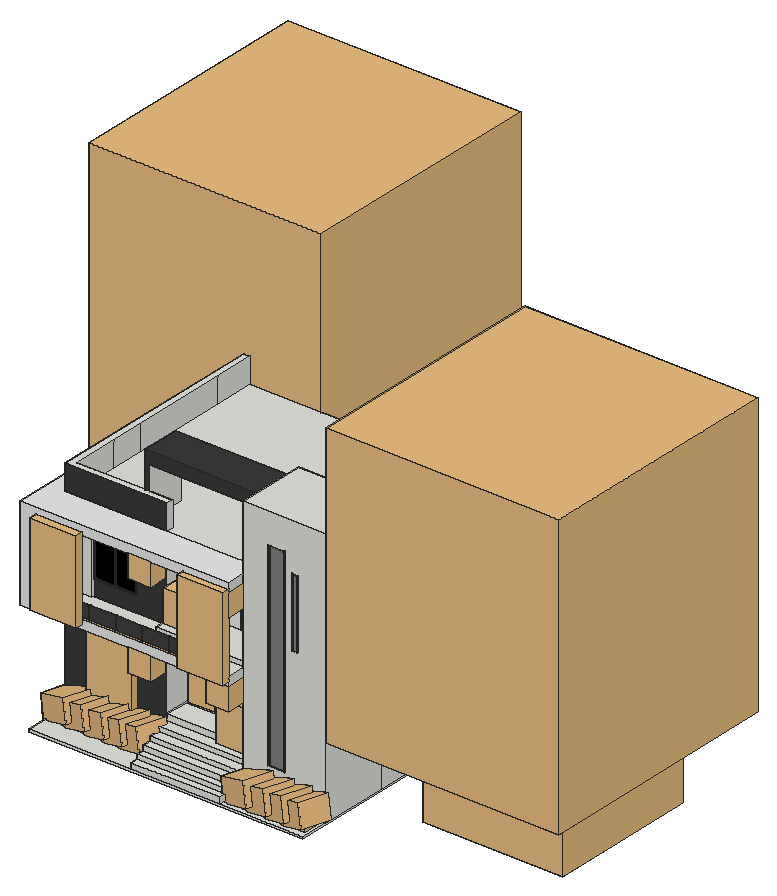
# SketchUp Ruby script. Lengths in inches.
U = 1.inch
M = Sketchup.active_model
def pt(a) = Geom::Point3d.new(a.map { |v| v * U })
def face(e, loops, mat)
  f = e.add_face(loops[0].map { |a| pt(a) })
  loops[1..].each { |l| e.add_face(l.map { |a| pt(a) }).erase! }
  f.material = f.back_material = mat if mat
  f
end
# faces: each face lists its corners as indices into pts; further lists are holes
def faces(e, pts, list, mat = nil) = list.each { |f| face(e, (f[0].is_a?(Array) ? f : [f]).map { |l| l.map { |i| pts[i] } }, mat) }
# xy, xz, yz: faces in a plane at the given z, y or x. An outline is a flat list of corners, or four numbers for a rectangle; further outlines are holes
def ring(l) = l.size == 4 ? [[l[0], l[1]], [l[2], l[1]], [l[2], l[3]], [l[0], l[3]]] : l.each_slice(2).to_a
def flat(e, list, mat, &to3) = list.each { |f| face(e, (f[0].is_a?(Array) ? f : [f]).map { |l| ring(l).map { |u, v| to3.(u, v) } }, mat) }
def xy(e, z, list, mat = nil) = flat(e, list, mat) { |x, y| [x, y, z] }
def xz(e, y, list, mat = nil) = flat(e, list, mat) { |x, z| [x, y, z] }
def yz(e, x, list, mat = nil) = flat(e, list, mat) { |y, z| [x, y, z] }
def lines(e, pts, list) = list.each { |a, b| e.add_line(pt(pts[a]), pt(pts[b])) }
# prism: a flat outline (further loops are holes) pulled along v
def prism(e, loops, v, mat = nil)
  f = face(e, loops, mat); d = Geom::Vector3d.new(v.map { |x| x * U })
  f.pushpull(f.normal.samedirection?(d) ? d.length : -d.length)
end
def box(e, o, s, mat = nil) = prism(e, [[o, [o[0] + s[0], o[1], o[2]], [o[0] + s[0], o[1] + s[1], o[2]], [o[0], o[1] + s[1], o[2]]]], [0, 0, s[2]], mat)
def at(x, y, z, deg = 0) = Geom::Transformation.translation(pt([x, y, z])) * Geom::Transformation.rotation(ORIGIN, Z_AXIS, deg.degrees)
def axes(o, x, y, z) = Geom::Transformation.new([*x, 0, *y, 0, *z, 0, *pt(o).to_a, 1])
def part(name) = M.definitions.add(name)
# library, detail: a bought-in or finely detailed component or shape, given as its bounding box
def library(name, o, s) = part(name).tap { |d| box(d.entities, o, s) }
def detail(e, o, s) = box(e.add_group.entities, o, s)
def put(e, d, t, mat = nil) = e.add_instance(d, t).tap { |i| i.material = mat if mat }
def group(e, t, mat = nil) = e.add_group.tap { |g| g.transformation = t; g.material = mat if mat }.entities
root = M.entities
M.materials.add("AM113_062_Tilia").color = [58, 81, 37]
M.materials.add("AM113_062_Tilia_Bark").color = [88, 85, 72]
M.materials.add("Glass_Tinted_Gray").color = [0, 0, 0]
M.materials.add("Material__1").color = [190, 136, 85]
M.materials.add("Material__2").color = [51, 42, 44]
M.materials.add("Material__3").color = [119, 136, 107]
M.materials.add("[0135_DarkGray]").color = [81, 81, 81]
M.materials.add("[Color M07]").color = [58, 58, 58]
M.materials.add("[Mirror 02]").color = [229, 229, 229]
M.materials.add("[Terrazzo Light Blue]").color = [196, 214, 227]
M.materials.add("[Translucent Glass Gray]1").color = [128, 128, 128]
M.materials.add("[Translucent_Glass_Blue]").color = [63, 63, 63]
M.materials.add("metal railing").color = [165, 165, 165]
M.materials.add("plastic2").color = [86, 86, 86]
M.materials.add("white_wall").color = [233, 233, 233]
c1 = library("PINTU+6+YA",[0,-0.6875,0],[35.83,8.07,80.71])
c2 = part("Window (2)")
xy(c2.entities,31.72,[[-0.78,88.6,2.72,128.1]])
xy(c2.entities,34.95,[[-0.78,91.53,0.84,106.59],[0.84,91.53,1.05,97.58],[1.05,91.53,1.42,106.59],[1.42,91.53,2.72,106.59],[0.84,97.58,1.05,98.18],
  [0.84,98.18,1.05,106.59]])
xy(c2.entities,35.27,[[-0.78,110.09,0.97,125.14],[1.05,110.09,2.72,125.14]])
xy(c2.entities,58.35,[[2.72,108.74,3.8,109.74]])
xy(c2.entities,77.8125,[[-0.78,110.09,2.72,125.14],[0.97,110.09,1.05,125.14]])
xy(c2.entities,77.93,[[-0.78,91.53,0.84,106.59],[1.05,91.53,1.42,106.59],[1.42,91.53,2.72,106.59]])
xy(c2.entities,80.72,[[-0.78,88.6,2.72,128.1]])
xz(c2.entities,88.6,[[-0.78,31.72,2.72,80.72]])
xz(c2.entities,91.53,[[-0.78,34.95,0.84,77.93],[1.05,34.95,1.42,77.93],[1.42,34.95,2.72,77.93]])
xz(c2.entities,106.59,[[-0.78,34.95,0.84,77.93],[0.84,34.95,1.05,77.93],[0.84,34.95,2.72,77.93]])
xz(c2.entities,108.74,[[3.8,54.35,4.22,54.6,4.22,59.47,2.72,59.97,2.72,58.35,3.8,58.35]])
xz(c2.entities,109.74,[[3.8,54.35,3.8,58.35,2.72,58.35,2.72,59.97,4.22,59.47,4.22,54.6]])
xz(c2.entities,110.09,[[-0.78,35.27,0.97,77.8125],[1.05,35.27,2.72,77.8125]])
xz(c2.entities,125.14,[[-0.78,35.27,0.97,77.8125],[0.97,35.27,1.05,80.72],[1.05,35.27,2.72,77.8125]])
xz(c2.entities,128.1,[[-0.78,31.72,2.72,80.72]])
yz(c2.entities,-0.78,[[[88.6,31.72,128.1,80.72],[91.53,34.95,106.59,77.93],[110.09,35.27,125.14,77.8125]]])
yz(c2.entities,0.84,[[91.53,34.95,106.59,77.93]])
yz(c2.entities,0.97,[[110.09,35.27,125.14,77.8125]])
yz(c2.entities,1.05,[[91.53,34.95,106.59,77.93],[110.09,35.27,125.14,77.8125]])
yz(c2.entities,1.42,[[91.53,34.95,106.59,77.93]])
yz(c2.entities,2.72,[[[88.6,31.72,108.35,80.72],[91.53,34.95,106.59,77.93]],[[108.35,31.72,128.1,80.72],[110.09,35.27,125.14,77.8125],[108.74,58.35,109.74,59.97]]])
yz(c2.entities,3.8,[[108.74,54.35,109.74,58.35]])
yz(c2.entities,4.22,[[108.74,54.6,109.74,59.47]])
# 4 loose lines left out
p = [[4.22,108.74,54.6],[3.8,108.74,54.35],[3.8,109.74,54.35],[4.22,109.74,54.6],[2.72,109.74,59.97],[2.72,108.74,59.97],
  [4.22,108.74,59.47],[4.22,109.74,59.47]]
faces(c2.entities,p,[[0,1,2,3],[4,5,6,7]])
c3 = part("PENTEK_RP Fineline 50S_Sliding_DoorCase_E1")
box(c3.entities,[0,0,0],[1.51,3.66,99.27],"[0135_DarkGray]")
c4 = part("PENTEK_RP Fineline 50S_SlidingDooe_Case_E2")
box(c4.entities,[0,0,0],[96.25,3.66,1.51],"[0135_DarkGray]")
c5 = part("pentek_RP Fineline 50S_SlidingDoor_Case")
put(c5.entities,c3,at(97.76,0,0))
put(c5.entities,c4,at(1.51,0,0))
put(c5.entities,c3,at(0,0,0))
put(c5.entities,c4,at(1.51,0,97.76))
c6 = part("PENTEK_RP Fineline 50S_SlidingDoor_GlazingBead_2")
box(c6.entities,[0,0,0],[0.56,0.59,94.39],"[0135_DarkGray]")
c7 = part("PENTEK_RP Fineline 50S_SlidingDoor_Glass")
box(c7.entities,[0,0,0],[46.58,0.16,94.39],"Glass_Tinted_Gray")
c8 = part("PENTEK_RP Fineline 50S_SlidingDoor_GlazingBead")
box(c8.entities,[0,0,0],[45.47,0.59,0.56],"[0135_DarkGray]")
c9 = part("PENTEK_RP Fineline 50S_SlidingDoor_Leaf_E1")
xy(c9.entities,0,[[0,0,0.93,1.97],[0.93,1.57,1.49,1.97]],"[0135_DarkGray]")
xy(c9.entities,96.25,[[0,0,0.93,0,0.93,1.57,1.49,1.57,1.49,1.97,0,1.97]],"[0135_DarkGray]")
xz(c9.entities,0,[[0,0,0.93,96.25]],"[0135_DarkGray]")
xz(c9.entities,1.57,[[0.93,0,1.49,95.32],[0.93,95.32,1.49,96.25]],"[0135_DarkGray]")
xz(c9.entities,1.97,[[0,0,1.49,96.25]],"[0135_DarkGray]")
yz(c9.entities,0,[[0,0,1.97,96.25]],"[0135_DarkGray]")
yz(c9.entities,0.93,[[0,0,1.57,0.93],[0,0.93,1.57,95.32],[0,95.32,1.57,96.25]],"[0135_DarkGray]")
yz(c9.entities,1.49,[[1.57,0,1.97,95.32],[1.57,95.32,1.97,96.25]],"[0135_DarkGray]")
c10 = part("PENTEK_RP Fineline 50S_SlidingDoor_Leaf_E2")
xy(c10.entities,0,[[0,0,0,1.57,0.56,1.57,0.56,1.97,46.02,1.97,46.02,1.57,46.58,1.57,46.58,0]],"[0135_DarkGray]")
xy(c10.entities,0.93,[[0,0,46.58,1.57]],"[0135_DarkGray]")
xy(c10.entities,1.49,[[0.56,1.57,46.02,1.97]],"[0135_DarkGray]")
xz(c10.entities,0,[[0,0,46.58,0.93]],"[0135_DarkGray]")
xz(c10.entities,1.57,[[0,0,0.56,0.93],[46.02,0,46.58,0.93],[0.56,0.93,46.02,1.49]],"[0135_DarkGray]")
xz(c10.entities,1.97,[[0.56,0,46.02,1.49]],"[0135_DarkGray]")
yz(c10.entities,0,[[0,0,1.57,0.93]],"[0135_DarkGray]")
yz(c10.entities,0.56,[[1.57,0,1.97,0.93],[1.57,0.93,1.97,1.49]],"[0135_DarkGray]")
yz(c10.entities,46.02,[[1.57,0,1.97,0.93],[1.57,0.93,1.97,1.49]],"[0135_DarkGray]")
yz(c10.entities,46.58,[[0,0,1.57,0.93]],"[0135_DarkGray]")
c11 = part("PENTEK_RP Fineline S_SlidingDoor_Leaf1")
put(c11.entities,c6,at(0.93,0,0.93))
put(c11.entities,c6,at(46.96,0,0.93))
put(c11.entities,c7,at(1.49,1.42,0.93))
put(c11.entities,c8,at(1.49,0,0.93))
put(c11.entities,c7,at(1.49,0.59,0.93),"[Terrazzo Light Blue]")
put(c11.entities,c9,at(0,0,0))
put(c11.entities,c9,axes([48.44,0,0],[-1,0,0],[0,1,0],[0,0,1]))
put(c11.entities,c10,axes([0.93,0,96.25],[1,0,0],[0,1,0],[0,0,-1]))
put(c11.entities,c10,at(0.93,0,0))
put(c11.entities,c8,at(1.49,0,94.77))
c12 = part("PENTEK_RP Fineline 50S_SlidingDoor_Leaf2")
put(c12.entities,c7,at(1.49,1.42,0.93))
put(c12.entities,c8,at(1.49,0,94.77))
put(c12.entities,c6,at(46.96,0,0.93))
put(c12.entities,c7,at(1.49,0.59,0.93),"[Mirror 02]")
put(c12.entities,c6,at(0.93,0,0.93))
put(c12.entities,c9,at(0,0,0))
put(c12.entities,c9,axes([48.44,0,0],[-1,0,0],[0,1,0],[0,0,1]))
put(c12.entities,c8,at(1.49,0,0.93))
put(c12.entities,c10,axes([0.93,0,96.25],[1,0,0],[0,1,0],[0,0,-1]))
put(c12.entities,c10,at(0.93,0,0))
c13 = part("PENTEK - Slimmest Steel Sliding Door / Window\#1")
put(c13.entities,c5,at(0,-1.88,-0.09))
put(c13.entities,c11,at(1.51,-2.27,1.42))
put(c13.entities,c12,at(49.32,-0.3,1.42))
c14 = library("Plante \#58",[-0.43,-1.58,0],[20.84,18.06,17.59])
c15 = library("Plant",[-21.8,-11.875,0],[94.69,106.42,111.78])
c16 = library("plant (1)",[-21.34,-27.21,-0.38],[41.91,41.15,38.97])
c17 = library("AM113_062_Tilia_Defintion",[-350.67,-364.73,-2.58],[672.29,726.36,1000])
c18 = library("AM113_062_Tilia_Defintion1",[-524.84,-500,219.37],[933.41,1000,877.77])
c19 = part("Group4\#1")
put(c19.entities,c17,axes([0,0,0],[0.28109,0,0],[0,0.28109,0],[0,0,0.28109]),"AM113_062_Tilia_Bark")
put(c19.entities,c18,axes([0,0,0],[0.33697,0,0],[0,0.33697,0],[0,0,0.33697]),"AM113_062_Tilia")
c20 = part("11")
put(c20.entities,c19,axes([-472.44,-237.95,314.96],[1,0,0],[0,0,-1],[0,1,0]))
c21 = library("\#2",[-119.83,-119.83,113.8],[239.66,239.66,17.4])
c22 = library("\#4",[-204.92,-212.35,-236.71],[424.28,257.5,472.53])
c23 = part("\#3")
put(c23.entities,c22,axes([-0.37,309.72,0],[1.36765,0,0],[0,1.36765,0],[0,0,1.36765]),"Material__3")
c24 = library("\#1",[-174.07,-174.07,0],[348.14,348.14,140])
c25 = part("9")
put(c25.entities,c21,at(-19.94,-24.66,0),"Material__2")
put(c25.entities,c23,axes([17.67,-32.6,40.29],[0.29694,0.9549,0],[-0.21403,0.06656,0.97456],[0.9306,-0.28939,0.22414]))
put(c25.entities,c24,at(-19.94,-24.66,0),"Material__1")
c26 = library("Railing",[0,0,0],[72,2.52,4.03])
c27 = part("railing plastic")
box(c27.entities,[0,0.75,0],[72,0.26,0.68],"plastic2")
box(c27.entities,[0,0,0],[72,0.26,0.68],"plastic2")
c28 = part("Glass Railing pro")
put(c28.entities,c26,axes([0,0,0],[7.25965,0,0],[0,1,0],[0,0,1]))
put(c28.entities,c27,axes([0,0.75,3.47],[7.25965,0,0],[0,1,0],[0,0,1]))
c29 = part("sheet glass")
box(c29.entities,[0,0,0],[39.37,0.39,39.37],"[Translucent_Glass_Blue]")
c30 = part("glass stretch")
box(c30.entities,[0,0,0],[39.37,0.39,43.31],"[Translucent_Glass_Blue]")
c31 = part("glass frame")
put(c31.entities,c29,axes([0,0,0],[1.8288,0,0],[0,1.016,0],[0,0,1]))
put(c31.entities,c30,axes([505.4,0,0],[0.43929,0,0],[0,1.016,0],[0,0,0.90909]))
put(c31.entities,c29,axes([72.2,0,0],[1.8288,0,0],[0,1.016,0],[0,0,1]))
put(c31.entities,c29,axes([144.4,0,0],[1.8288,0,0],[0,1.016,0],[0,0,1]))
put(c31.entities,c29,axes([216.6,0,0],[1.8288,0,0],[0,1.016,0],[0,0,1]))
put(c31.entities,c29,axes([288.8,0,0],[1.8288,0,0],[0,1.016,0],[0,0,1]))
put(c31.entities,c29,axes([361,0,0],[1.8288,0,0],[0,1.016,0],[0,0,1]))
put(c31.entities,c29,axes([433.2,0,0],[1.8288,0,0],[0,1.016,0],[0,0,1]))
c32 = part("Glass Railing +")
put(c32.entities,c28,at(0,0,0),"metal railing")
put(c32.entities,c31,at(0,1.0625,1.53),"metal railing")
c33 = part("My+Glass_Railing")
put(c33.entities,c32,at(-0.34,0,0))
c34 = library("Shrub+_Grass",[-121.83,-22.34,0],[123.96,19.94,123.95])
xy(root,1.25,[[323.61,0,323.61,121.6875,46.9375,121.6875,46.9375,725.65,788.76,725.65,788.76,76.875,564.05,76.875,564.05,0]])
xy(root,17.91,[[323.61,0,564.05,19.6875]])
xy(root,28.84,[[323.61,19.6875,564.05,40.375]])
xy(root,42.15,[[323.61,40.375,564.05,64.0625]])
xy(root,54.11,[[323.61,64.0625,564.05,89.1875]])
xy(root,66.27,[[323.61,89.1875,564.05,121.6875]])
xy(root,80.94,[[323.61,121.6875,564.05,187.1875]])
xy(root,84,[[633.22,76.875,678.12,143.25]])
xy(root,84.75,[[327.13,187.1875,401.74,220.1875]])
xy(root,94.03,[[426.44,187.1875,555.82,205.0625]])
xy(root,105.22,[[124.34,121.6875,241.78,148.5625]])
xy(root,109.98,[[46.9375,151.95,78.125,247.52]])
xy(root,115.22,[[46.9375,435.18,88.75,569.75]])
xy(root,249.78,[[124.34,121.6875,241.78,148.5625],[46.9375,151.95,78.125,247.52],[327.13,187.1875,401.74,220.1875],[426.44,187.1875,555.82,205.0625],[46.9375,435.18,88.75,569.75]])
xy(root,273.04,[[0,28.625,0,278.26,46.9375,278.26,46.9375,121.6875,323.61,121.6875,323.61,187.1875,564.05,187.1875,564.05,28.625]],"white_wall")
xy(root,297.35,[[41.45,28.625,564.05,28.625,564.05,83.29,323.61,83.29,323.61,121.6875,124.34,121.6875,124.34,115.3125,46.9375,115.3125,46.9375,278.26,13.75,278.26,13.75,130.3125,18.45,130.3125,18.45,82.67,41.45,82.67],[46.9375,115.3125,124.34,121.6875],[0,130.3125,10.1875,278.26],[10.1875,130.3125,13.75,278.26]])
xy(root,308.91,[[323.61,83.29,564.05,83.29,564.05,187.1875,555.82,187.1875,555.82,207.4375,469.9,207.4375,469.9,187.1875,323.61,187.1875]])
xy(root,336.96,[[46.9375,422.72,118.5,567.03]])
xy(root,339.36,[[124.34,121.6875,241.78,141.4375]])
xy(root,364.43,[[376.875,187.1875,463.375,205.25]])
xy(root,385.18,[[697.23,76.875,713.16,135.5625]])
xy(root,457.89,[[124.34,121.6875,241.78,141.4375]])
xy(root,469.24,[[376.875,187.1875,463.375,205.25],[469.9,187.1875,555.82,207.4375]])
xy(root,481.27,[[46.9375,422.72,118.5,567.03]])
xy(root,500.91,[[46.9375,115.3125,124.34,121.6875],[0,130.3125,10.1875,278.26],[10.1875,130.3125,13.75,278.26]])
xy(root,500.91,[[41.45,28.625,41.45,82.67,18.45,82.67,18.45,130.3125,13.75,130.3125,13.75,278.26,46.9375,278.26,46.9375,115.3125,124.34,115.3125,124.34,121.6875,323.61,121.6875,323.61,187.1875,564.05,187.1875,564.05,28.625],[0,353.16,46.9375,615.47]],"white_wall")
xy(root,525.1,[[323.61,121.6875,564.05,121.6875,564.05,725.65,65.125,725.65,65.125,139.5,250.55,139.5,250.55,242.3125,264.05,242.3125,264.05,139.5,323.61,139.5],[564.05,265.5,788.76,725.65]])
xy(root,525.1,[[0,28.625,564.05,28.625,564.05,121.6875,46.9375,121.6875,46.9375,278.26,0,278.26],[0,353.16,46.9375,615.47]],"white_wall")
xy(root,573.56,[[697.23,76.875,713.16,135.5625]])
xy(root,592.47,[[46.9375,121.6875,323.61,121.6875,323.61,139.5,65.125,139.5,65.125,725.65,46.9375,725.65]])
xy(root,620.81,[[633.22,76.875,678.12,143.25]])
xy(root,656.55,[[264.05,139.5,564.05,242.3125]],"[Color M07]")
xy(root,690.29,[[250.55,139.5,564.05,242.3125]],"[Color M07]")
xy(root,701.22,[[564.05,76.875,788.76,265.5]])
xz(root,0,[[323.61,1.25,564.05,17.91]])
xz(root,19.6875,[[323.61,17.91,564.05,28.84]])
xz(root,28.625,[[0,273.04,564.05,273.04,564.05,297.35,41.45,297.35,41.45,500.91,564.05,500.91,564.05,525.1,0,525.1]],"white_wall")
xz(root,40.375,[[323.61,28.84,564.05,42.15]])
xz(root,64.0625,[[323.61,42.15,564.05,54.11]])
xz(root,76.875,[[[564.05,1.25,788.76,701.22],[633.22,84,678.12,620.81],[697.23,385.18,713.16,573.56]]])
xz(root,82.67,[[18.45,297.35,41.45,500.91]])
xz(root,83.29,[[323.61,297.35,564.05,308.91]])
xz(root,89.1875,[[323.61,54.11,564.05,66.27]])
xz(root,115.3125,[[46.9375,297.35,124.34,500.91]])
xz(root,121.6875,[[323.61,66.27,564.05,80.94],[124.34,273.04,241.78,297.35],[46.9375,297.35,124.34,500.91],[46.9375,500.91,323.61,525.1]])
xz(root,121.6875,[[[46.9375,1.25,323.61,273.04],[124.34,105.22,241.78,249.78]],[124.34,297.35,323.61,297.35,323.61,500.91,124.34,500.91,124.34,457.89,241.78,457.89,241.78,339.36,124.34,339.36],[46.9375,525.1,323.61,592.47]],"[Color M07]")
xz(root,130.3125,[[0,297.35,10.1875,500.91],[10.1875,297.35,13.75,500.91],[13.75,297.35,18.45,500.91]])
xz(root,135.5625,[[697.23,385.18,713.16,573.56]])
xz(root,139.5,[[65.125,525.1,250.55,592.47],[264.05,525.1,323.61,592.47]])
xz(root,139.5,[[250.55,592.47,264.05,592.47,264.05,656.55,564.05,656.55,564.05,690.29,250.55,690.29]],"[Color M07]")
xz(root,141.4375,[[124.34,339.36,241.78,457.89]])
xz(root,143.25,[[633.22,84,678.12,620.81]])
xz(root,148.5625,[[124.34,105.22,241.78,249.78]])
xz(root,151.95,[[46.9375,109.98,78.125,249.78]])
xz(root,187.1875,[[323.61,80.94,564.05,84.75]])
xz(root,187.1875,[[323.61,84.75,327.13,84.75,327.13,249.78,401.74,249.78,401.74,84.75,426.44,84.75,426.44,273.04,323.61,273.04],[426.44,84.75,564.05,84.75,564.05,273.04,426.44,273.04,426.44,249.78,555.82,249.78,555.82,94.03,426.44,94.03],[323.61,308.91,469.9,308.91,469.9,469.24,463.375,469.24,463.375,364.43,376.875,364.43,376.875,469.24,555.82,469.24,555.82,308.91,564.05,308.91,564.05,500.91,323.61,500.91]],"white_wall")
xz(root,205.0625,[[426.44,94.03,555.82,249.78]])
xz(root,205.25,[[376.875,364.43,463.375,469.24]])
xz(root,207.4375,[[469.9,308.91,555.82,469.24]])
xz(root,220.1875,[[327.13,84.75,401.74,249.78]])
xz(root,242.3125,[[250.55,525.1,250.55,690.29,564.05,690.29,564.05,656.55,264.05,656.55,264.05,525.1]])
xz(root,247.52,[[46.9375,109.98,78.125,249.78]])
xz(root,265.5,[[564.05,525.1,788.76,701.22]])
xz(root,278.26,[[0,273.04,46.9375,297.35],[10.1875,297.35,13.75,500.91],[0,500.91,46.9375,525.1]])
xz(root,353.16,[[0,500.91,46.9375,525.1]],"white_wall")
xz(root,422.72,[[46.9375,336.96,118.5,481.27]])
xz(root,435.18,[[46.9375,115.22,88.75,249.78]])
xz(root,567.03,[[46.9375,336.96,118.5,481.27]])
xz(root,569.75,[[46.9375,115.22,88.75,249.78]])
xz(root,615.47,[[0,500.91,46.9375,525.1]])
xz(root,725.65,[[46.9375,1.25,788.76,84.75],[46.9375,84.75,788.76,273.04],[46.9375,273.04,788.76,297.35],[46.9375,297.35,46.9375,500.91,564.05,500.91,564.05,525.1,788.76,525.1,788.76,297.35],[46.9375,500.91,46.9375,592.47,65.125,592.47,65.125,525.1,564.05,525.1,564.05,500.91]])
yz(root,0,[[28.625,273.04,28.625,525.1,278.26,525.1,278.26,500.91,130.3125,500.91,130.3125,297.35,278.26,297.35,278.26,273.04],[353.16,500.91,615.47,525.1]],"white_wall")
yz(root,10.1875,[[130.3125,297.35,278.26,500.91]])
yz(root,13.75,[[130.3125,297.35,278.26,500.91]])
yz(root,18.45,[[82.67,297.35,130.3125,500.91]])
yz(root,41.45,[[28.625,297.35,82.67,500.91]])
yz(root,46.9375,[[121.6875,1.25,725.65,84.75],[115.3125,297.35,121.6875,500.91],[121.6875,500.91,278.26,525.1],[353.16,500.91,615.47,525.1]])
yz(root,46.9375,[[[121.6875,84.75,121.6875,273.04,278.26,273.04,278.26,297.35,121.6875,297.35,121.6875,500.91,278.26,500.91,278.26,525.1,121.6875,525.1,121.6875,592.47,725.65,592.47,725.65,84.75],[422.72,336.96,567.03,481.27],[435.18,115.22,569.75,249.78],[151.95,109.98,247.52,249.78],[353.16,500.91,615.47,525.1]]],"[Color M07]")
yz(root,65.125,[[139.5,525.1,266.01,592.47],[266.01,525.1,353.16,592.47],[353.16,525.1,615.47,592.47],[615.47,525.1,725.65,592.47]])
yz(root,78.125,[[151.95,109.98,247.52,249.78]])
yz(root,88.75,[[435.18,115.22,569.75,249.78]])
yz(root,118.5,[[422.72,336.96,567.03,481.27]])
yz(root,124.34,[[121.6875,105.22,148.5625,249.78],[115.3125,297.35,121.6875,500.91],[121.6875,339.36,141.4375,457.89]])
yz(root,241.78,[[121.6875,105.22,148.5625,249.78],[121.6875,339.36,141.4375,457.89]])
yz(root,250.55,[[139.5,525.1,242.3125,690.29]],"[Color M07]")
yz(root,264.05,[[139.5,525.1,242.3125,656.55]])
yz(root,323.61,[[0,1.25,0,17.91,19.6875,17.91,19.6875,28.84,40.375,28.84,40.375,42.15,64.0625,42.15,64.0625,54.11,89.1875,54.11,89.1875,66.27,121.6875,66.27,121.6875,1.25],[121.6875,80.94,187.1875,84.75],[121.6875,84.75,187.1875,273.04],[83.29,297.35,121.6875,308.91],[121.6875,308.91,187.1875,500.91],
  [121.6875,525.1,139.5,592.47]])
yz(root,327.13,[[187.1875,84.75,220.1875,249.78]])
yz(root,376.875,[[187.1875,364.43,205.25,469.24]])
yz(root,401.74,[[187.1875,84.75,220.1875,249.78]])
yz(root,426.44,[[187.1875,94.03,205.0625,249.78]])
yz(root,463.375,[[187.1875,364.43,205.25,469.24]])
yz(root,469.9,[[187.1875,308.91,207.4375,469.24]])
yz(root,555.82,[[187.1875,94.03,205.0625,249.78],[187.1875,308.91,207.4375,469.24]])
yz(root,564.05,[[0,1.25,76.875,1.25,76.875,54.11,64.0625,54.11,64.0625,42.15,40.375,42.15,40.375,28.84,19.6875,28.84,19.6875,17.91,0,17.91],[76.875,54.11,76.875,84.75,187.1875,84.75,187.1875,80.94,121.6875,80.94,121.6875,66.27,89.1875,66.27,89.1875,54.11],[76.875,84.75,187.1875,273.04],[28.625,273.04,76.875,297.35],[76.875,297.35,76.875,500.91,187.1875,500.91,187.1875,308.91,83.29,308.91,83.29,297.35],
  [28.625,500.91,76.875,525.1],[76.875,500.91,160.1875,525.1],[160.1875,500.91,725.65,525.1],[[76.875,525.1,265.5,701.22],[139.5,656.55,242.3125,690.29]]])
yz(root,633.22,[[76.875,84,143.25,620.81]])
yz(root,678.12,[[76.875,84,143.25,620.81]])
yz(root,697.23,[[76.875,385.18,135.5625,573.56]])
yz(root,713.16,[[76.875,385.18,135.5625,573.56]])
yz(root,788.76,[[76.875,1.25,265.5,701.22],[265.5,1.25,725.65,525.1]])
# 1 loose lines left out
put(root,c1,axes([327.13,187.1875,84.75],[2.08229,0,0],[0,1,0],[0,0,2.04476]))
put(root,c1,axes([469.9,187.1875,308.91],[2.3979,0,0],[0,1,0],[0,0,1.9865]))
put(root,c2,axes([49.38,136.98,29.29],[3.1248,0,0],[0,3.37197,0],[0,0,2.72326]))
put(root,c2,axes([49.38,100.07,244.3],[3.1248,0,0],[0,3.64173,0],[0,0,2.91389]))
put(root,c13,axes([124.34,123.56,339.47],[1.18298,0,0],[0,1,0],[0,0,1.194]))
put(root,c13,axes([124.34,123.56,105.35],[1.18298,0,0],[0,1,0],[0,0,1.45622]))
put(root,c13,axes([426.44,189.33,94.17],[1.30323,0,0],[0,1,0],[0,0,1.56892]))
put(root,c13,axes([376.875,190.01,362.65],[0.87134,0,0],[0,0.62,0],[0,0,1.07472]))
put(root,c14,axes([291.9375,32.98,211.83],[2.9928,0,0],[0,2.7666,0],[0,0,3.48]))
put(root,c14,axes([502.97,32.98,211.83],[2.9928,0,0],[0,2.7666,0],[0,0,3.48]))
put(root,c14,axes([291.9375,32.98,439.71],[2.9928,0,0],[0,2.7666,0],[0,0,3.48]))
put(root,c14,axes([502.97,32.98,439.71],[2.9928,0,0],[0,2.7666,0],[0,0,3.48]))
put(root,c15,at(503.1,101.8125,80.94))
put(root,c16,axes([368.15,160.01,309.75],[2.0178,0,0],[0,1.9494,0],[0,0,2.1888]))
put(root,c20,axes([2087.36,1043.77,617.04],[2,0,0],[0,0,2.58],[0,-2,0]))
put(root,c25,axes([758.16,43.88,-2.35],[0.1342,0,0],[0,0.1342,0],[0,0,0.17849]))
put(root,c25,axes([663.72,43.88,-2.35],[0.1342,0,0],[0,0.1342,0],[0,0,0.17849]))
put(root,c25,axes([609.41,43.88,-2.35],[0.1342,0,0],[0,0.1342,0],[0,0,0.17849]))
put(root,c25,axes([712.91,43.88,-2.35],[0.1342,0,0],[0,0.1342,0],[0,0,0.17849]))
put(root,c33,at(41.69,28.625,297.35))
put(root,c34,axes([561.92,31.03,284.22],[1,0,0],[0,1,0],[0,0,1.815]))
put(root,c34,axes([165.74,31.03,284.22],[1,0,0],[0,1,0],[0,0,1.815]))
put(root,c34,axes([240.37,125,43],[1,0,0],[0,1,0],[0,0,1.815]))
put(root,c2,axes([49.38,-67.59,21.94],[3.1248,0,0],[0,2.46154,0],[0,0,2.80496]))
put(root,c20,axes([926.73,1692.54,617.04],[2,0,0],[0,0,2.58],[0,-2,0]))
g1 = group(root,at(633.22,76.875,84))
xy(g1,0,[[0,0,44.9,1.875]],"[Color M07]")
xy(g1,3.09,[[3.09,0,41.81,1.875]],"[Color M07]")
xy(g1,533.72,[[3.09,0,41.81,1.875]],"[Color M07]")
xy(g1,536.8125,[[0,0,44.9,1.875]],"[Color M07]")
xz(g1,0,[[[0,0,44.9,536.8125],[3.09,3.09,41.81,533.72]]],"[Color M07]")
xz(g1,0,[[3.09,3.09,41.81,533.72]],"[Translucent Glass Gray]1")
xz(g1,1.875,[[[0,0,44.9,536.8125],[3.09,3.09,41.81,533.72]]],"[Color M07]")
yz(g1,0,[[0,0,1.875,536.8125]],"[Color M07]")
yz(g1,3.09,[[0,3.09,1.875,533.72]],"[Color M07]")
yz(g1,41.81,[[0,3.09,1.875,533.72]],"[Color M07]")
yz(g1,44.9,[[0,0,1.875,536.8125]],"[Color M07]")
g2 = group(root,at(697.23,76.875,385.18),"[Color M07]")
xy(g2,0,[[0,0,15.93,0.25]],"[Color M07]")
xy(g2,1.75,[[1.75,0,14.18,0.25]],"[Color M07]")
xy(g2,186.62,[[1.75,0,14.18,0.25]],"[Color M07]")
xy(g2,188.375,[[0,0,15.93,0.25]],"[Color M07]")
xz(g2,0,[[[0,0,15.93,188.375],[1.75,1.75,14.18,186.62]]],"[Color M07]")
xz(g2,0,[[1.75,1.75,14.18,186.62]],"[Translucent Glass Gray]1")
xz(g2,0.25,[[[0,0,15.93,188.375],[1.75,1.75,14.18,186.62]]],"[Color M07]")
yz(g2,0,[[0,0,0.25,188.375]],"[Color M07]")
yz(g2,1.75,[[0,1.75,0.25,186.62]],"[Color M07]")
yz(g2,14.18,[[0,1.75,0.25,186.62]],"[Color M07]")
yz(g2,15.93,[[0,0,0.25,188.375]],"[Color M07]")
g3 = group(root,at(46.9375,725.65,-36.1875))
box(g3,[0,-725.65,31.4375],[741.82,725.65,6])
g4 = group(root,at(46.28,40.73,-2.35))
put(g4,c25,axes([239.2,45.89,0],[0.1342,0,0],[0,0.1342,0],[0,0,0.17849]))
put(g4,c25,axes([144.76,45.89,0],[0.1342,0,0],[0,0.1342,0],[0,0,0.17849]))
put(g4,c25,axes([90.45,45.89,0],[0.1342,0,0],[0,0.1342,0],[0,0,0.17849]))
put(g4,c25,axes([193.95,45.89,0],[0.1342,0,0],[0,0.1342,0],[0,0,0.17849]))
put(g4,c25,axes([42.2,45.89,0],[0.1342,0,0],[0,0.1342,0],[0,0,0.17849]))
